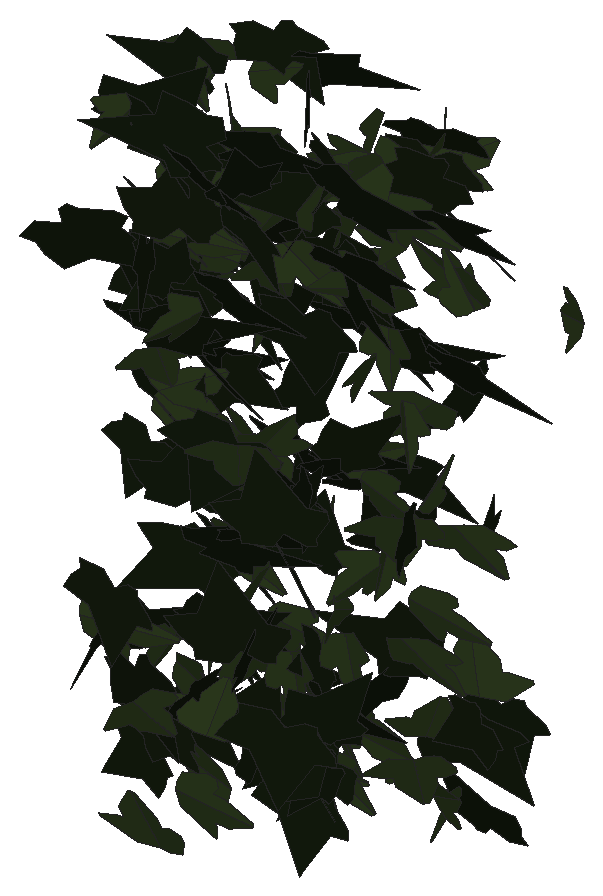
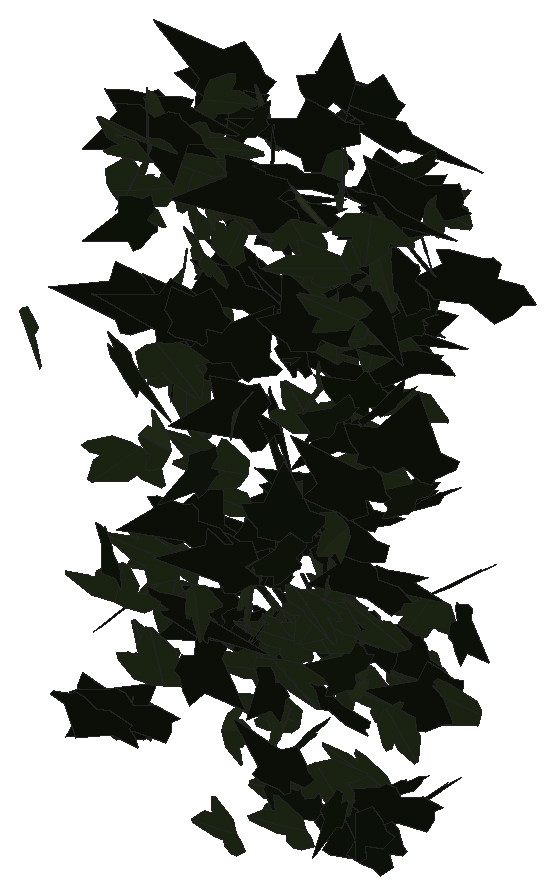
# SketchUp Ruby script. Lengths in millimetres.
U = 1.mm
M = Sketchup.active_model
def pt(a) = Geom::Point3d.new(a.map { |v| v * U })
def face(e, loops, mat)
  f = e.add_face(loops[0].map { |a| pt(a) })
  loops[1..].each { |l| e.add_face(l.map { |a| pt(a) }).erase! }
  f.material = f.back_material = mat if mat
  f
end
# faces: each face lists its corners as indices into pts; further lists are holes
def faces(e, pts, list, mat = nil) = list.each { |f| face(e, (f[0].is_a?(Array) ? f : [f]).map { |l| l.map { |i| pts[i] } }, mat) }
# xy, xz, yz: faces in a plane at the given z, y or x. An outline is a flat list of corners, or four numbers for a rectangle; further outlines are holes
def ring(l) = l.size == 4 ? [[l[0], l[1]], [l[2], l[1]], [l[2], l[3]], [l[0], l[3]]] : l.each_slice(2).to_a
def flat(e, list, mat, &to3) = list.each { |f| face(e, (f[0].is_a?(Array) ? f : [f]).map { |l| ring(l).map { |u, v| to3.(u, v) } }, mat) }
def xy(e, z, list, mat = nil) = flat(e, list, mat) { |x, y| [x, y, z] }
def xz(e, y, list, mat = nil) = flat(e, list, mat) { |x, z| [x, y, z] }
def yz(e, x, list, mat = nil) = flat(e, list, mat) { |y, z| [x, y, z] }
def lines(e, pts, list) = list.each { |a, b| e.add_line(pt(pts[a]), pt(pts[b])) }
# prism: a flat outline (further loops are holes) pulled along v
def prism(e, loops, v, mat = nil)
  f = face(e, loops, mat); d = Geom::Vector3d.new(v.map { |x| x * U })
  f.pushpull(f.normal.samedirection?(d) ? d.length : -d.length)
end
def box(e, o, s, mat = nil) = prism(e, [[o, [o[0] + s[0], o[1], o[2]], [o[0] + s[0], o[1] + s[1], o[2]], [o[0], o[1] + s[1], o[2]]]], [0, 0, s[2]], mat)
def at(x, y, z, deg = 0) = Geom::Transformation.translation(pt([x, y, z])) * Geom::Transformation.rotation(ORIGIN, Z_AXIS, deg.degrees)
def axes(o, x, y, z) = Geom::Transformation.new([*x, 0, *y, 0, *z, 0, *pt(o).to_a, 1])
def part(name) = M.definitions.add(name)
# library, detail: a bought-in or finely detailed component or shape, given as its bounding box
def library(name, o, s) = part(name).tap { |d| box(d.entities, o, s) }
def detail(e, o, s) = box(e.add_group.entities, o, s)
def put(e, d, t, mat = nil) = e.add_instance(d, t).tap { |i| i.material = mat if mat }
def group(e, t, mat = nil) = e.add_group.tap { |g| g.transformation = t; g.material = mat if mat }.entities
root = M.entities
M.materials.add("efeu1").color = [18, 25, 13]
M.materials.add("efeu2").color = [43, 57, 29]
c1 = part("ivyleaf_10")
p = [[0,12.8,-0.8],[-1.5,51.3,-10.9],[-4.9,51,-11.6],[-13.6,26.5,-7.3],[-13.2,15.9,-4.6],[-21.1,19.3,-7.2],
  [-29.5,16.3,-8.3],[-29.2,8.3,-6.2],[-19.7,-9.8,0.5],[-7.6,-13,4],[1,-12.2,5.8],[-0.4,51.1,-11.1],
  [-1.5,51.1,-10.9],[1,-12.4,5.9],[16.9,-12.4,3.5],[35.1,9.1,-5.1],[35,12.9,-6.1],[20.5,16.4,-4.9],
  [15.8,15,-3.8],[15.3,27.6,-7.1],[12.8,31.3,-7.8]]
faces(c1.entities,p,[[0,1,2,3,4,5,6,7,8,9,10],[11,12,0,13,14,15,16,17,18,19,20]],"efeu2")
c2 = part("ivyleaf_9")
p = [[39.1,54.8,31.7],[34.5,51.8,30.2],[-5.3,25.2,17.3],[-17.9,28.3,20.9],[-21.6,21.7,17],[-20.2,4.3,5.3],
  [-22.9,-0.3,2.5],[-17.1,-4,-0.6],[-2,-2.1,-1.2],[-0.7,-15.4,-10.1],[16.6,-22.3,-16.7],[21.1,-15.1,-12.5],
  [32.7,-10.7,-11],[46.1,-1.8,-6.6],[30.8,11.2,3.8]]
faces(c2.entities,p,[[0,1,2,3,4,5,6,7,8,9,10,11,12,13,14]],"efeu1")
put(root,c1,axes([4846,848.6,1966.5],[1.18258,-0.23138,-0.81582],[1.49962,-0.21628,0.66148],[-0.59651,-1.00243,0.04559]))
put(root,c1,axes([4885.7,700.2,2538.1],[-0.36711,-0.69452,0.88742],[0.07213,-0.90382,-0.69911],[2.14348,-0.08853,0.17551]))
put(root,c1,axes([4836.3,714.6,1809.9],[0.3187,-0.20437,-1.17963],[2.21627,-0.24872,0.2084],[-0.52897,-1.16521,0.16242]))
put(root,c2,axes([4878.1,784.3,2193.3],[2.14412,-0.25981,0.56554],[-1.04967,0.1251,1.15616],[-0.5488,-1.25434,-0.00183]))
put(root,c2,axes([4866.7,834.1,1632.7],[0.89169,0.91791,0.16625],[-0.1858,-0.13677,1.03028],[1.76564,-0.47796,0.02446]))
put(root,c2,axes([4851.8,797,2484.4],[0.18117,0.02377,-1.09498],[2.08435,-0.01319,0.09492],[-0.02109,-1.09903,-0.02482]))
put(root,c2,axes([4929.7,790.7,2565.8],[-1.03003,0.34094,0.81684],[-1.45047,0.30741,-0.63327],[-0.85671,-0.93039,0.09008]))
put(root,c1,axes([4893.3,836.9,2570],[-1.65299,-0.58891,-0.0854],[0.14393,0.04063,-1.04933],[1.12335,-0.87177,0.00879]))
put(root,c2,axes([4905,802.3,2267.8],[-0.88881,-0.81019,0.7348],[0.6949,0.63767,0.93514],[-1.96226,0.5928,-0.00167]))
put(root,c2,axes([4867.5,714.2,1803.7],[0.4301,0.19051,1.17744],[1.81265,0.6926,-0.29486],[-1.36655,0.97865,-0.02054]))
put(root,c1,axes([4901.7,773.6,1792.3],[-0.28561,-1.14491,0.34896],[-0.0254,-0.35007,-1.15429],[2.27782,-0.14746,0.03088]))
put(root,c2,axes([4860.8,618.8,2404.9],[0.2146,0.04854,-1.35483],[0.99531,1.25272,0.08841],[2.38046,-0.52816,0.08517]))
put(root,c1,axes([4905.7,792.9,2483.9],[-0.23456,-1.0959,-0.05158],[0.01073,0.05127,-1.10281],[2.088,-0.12337,-0.00013]))
put(root,c2,axes([4897.8,894.6,1717.6],[1.17847,-0.34894,-0.75473],[-1.18072,0.43266,-0.70903],[1.05366,0.87512,0.04961]))
put(root,c2,axes([4899.7,725.4,1645.2],[0.56188,-0.65632,-0.84207],[0.61853,-0.77696,0.71952],[-1.93548,-0.43883,-0.01452]))
put(root,c2,axes([4876.7,763.3,2131],[0.64432,-0.96981,0.40729],[0.38099,-0.36064,-1.02513],[1.96532,0.38786,0.0652]))
put(root,c2,axes([4887.9,782.7,1681.3],[-0.24413,-0.55305,-1.09213],[0.4735,1.06342,-0.56773],[2.28124,-0.27991,0.00096]))
put(root,c2,axes([4915.4,621.2,1867.1],[-0.76393,0.48456,-0.93814],[1.18497,-0.70197,-0.62897],[-1.62302,-0.74058,-0.01765]))
put(root,c2,axes([4881.4,745.3,2394],[1.04099,-0.82406,0.44768],[0.46426,-0.3754,-0.98906],[1.7234,0.59889,-0.00397]))
put(root,c2,axes([4915.5,707.1,2085],[-0.61667,-0.93712,0.43634],[-0.30194,-0.40677,-0.99143],[1.94407,-0.36044,-0.01557]))
put(root,c2,axes([4885.1,861.7,1651],[0.46559,-0.58363,0.86638],[1.32845,-0.5707,-0.58154],[1.47916,0.69626,0.24958]))
put(root,c1,axes([4907.7,796.2,2558.5],[-0.7182,0.19841,-0.94224],[0.76416,-0.88741,-0.34767],[-1.66567,-0.49267,0.24677]))
put(root,c2,axes([4952.8,775.8,2416.3],[0.70779,0.07914,-1.04316],[-1.96269,-0.15844,-0.37967],[-0.33481,1.09607,0.02043]))
put(root,c2,axes([4911.5,740.5,1678.1],[0.52368,-0.71599,-0.67061],[-0.28279,0.65804,-0.76353],[1.8455,0.304,0.0733]))
put(root,c2,axes([4907.6,707.4,2529.9],[-1.02548,-0.17609,1.14757],[2.17278,0.14966,0.559],[-0.40173,1.2589,0.09406]))
put(root,c2,axes([4900.4,816,2023.8],[-0.26356,-0.22747,-1.05466],[1.65883,0.60312,-0.24453],[1.21025,-0.87621,0.10548]))
put(root,c1,axes([4950.4,863.7,1733.6],[-0.95398,-0.91522,0.38623],[-0.31352,-0.35004,-1.04326],[1.86443,-0.52716,0.02219]))
put(root,c2,axes([4927.5,623.3,1922.4],[-0.37026,-1.21348,0.33962],[-0.11374,-0.33437,-1.22896],[2.39553,-0.20343,-0.00586]))
put(root,c1,axes([4940.5,693.8,2224.6],[-1.0711,-0.94475,-0.38083],[0.42097,0.31136,-1.09929],[1.89238,-0.604,0.02899]))
put(root,c2,axes([4910.8,850.8,1893.8],[0.96676,-0.90302,0.37203],[0.34876,-0.32377,-1.03609],[1.82576,0.54001,0.00092]))
put(root,c2,axes([4934.1,729,2314.2],[-1.14695,-0.91496,-0.60108],[0.62428,0.5037,-1.09559],[1.98777,-0.68612,-0.00274]))
put(root,c2,axes([4913,829.8,2149.9],[1.8282,0.40208,-0.31312],[0.55286,0.11694,1.04134],[0.79691,-1.00355,-0.00411]))
put(root,c1,axes([4960.3,886.9,2004.7],[1.67581,-0.45234,-0.39639],[-0.65056,0.20187,-0.98968],[0.94182,0.9443,0.02169]))
put(root,c2,axes([4995,729.9,2335.6],[-1.34925,0.01881,0.95009],[-1.80656,-0.06991,-0.7069],[0.08528,-1.18337,0.05687]))
put(root,c2,axes([4945.7,740,2503.9],[-0.77998,-1.09276,-0.27634],[0.19264,0.25717,-1.16707],[2.13653,-0.42212,0.00435]))
put(root,c1,axes([4974.5,917.2,1908.8],[1.82703,-0.05891,-0.44476],[-0.84624,0.01509,-0.96172],[0.1138,1.05789,-0.01105]))
put(root,c1,axes([4940,824.2,2412],[0.83206,0.37666,-0.93166],[1.36345,0.59568,0.57701],[1.34123,-0.83922,-0.00859]))
put(root,c1,axes([4996.9,735.4,1635.3],[0.10107,-0.03825,-1.11885],[-1.45993,0.81459,-0.06426],[1.55186,0.76883,0.01242]))
put(root,c1,axes([4967.5,727.3,2337.2],[-1.56086,-0.69456,-0.20292],[0.28902,0.13467,-1.07471],[1.34648,-0.83406,-0.00455]))
put(root,c1,axes([4956.2,823.4,2081.1],[-1.21348,0.84104,-0.32874],[0.3791,-0.26153,-1.05541],[-1.67627,-0.66799,-0.0007]))
put(root,c2,axes([4991.7,702.2,2348.9],[-1.84264,-0.54092,0.3383],[-0.52851,-0.19624,-1.10851],[1.09319,-1.00663,0.03431]))
put(root,c2,axes([4998,714.2,1951.4],[-1.9086,-0.47753,0.46517],[-0.77208,-0.22963,-1.11031],[1.0068,-1.08136,0.03037]))
put(root,c2,axes([5007.5,653.9,2303],[0.35354,-0.22916,1.33655],[-1.51332,1.07437,0.29472],[-2.09059,-0.81646,0.01268]))
put(root,c1,axes([4966.9,840.5,1964.7],[-1.62663,-0.48057,-0.40885],[0.65443,0.2224,-0.98024],[1.00683,-0.92096,-0.02338]))
put(root,c1,axes([4941.8,720.7,2167.5],[1.36561,0.02191,-0.77898],[1.47716,0.07501,0.71703],[0.1332,-1.05643,0.03476]))
put(root,c2,axes([4950.5,680.1,2552.1],[0.34669,-1.10973,0.43678],[0.21296,-0.42399,-1.12391],[2.25973,0.21021,0.03891]))
put(root,c1,axes([5010.2,724.9,2370.8],[0.366,0.1832,1.06547],[-1.68571,-0.59383,0.26197],[1.1798,-0.9053,0.04378]))
put(root,c1,axes([4961,738.4,2426.1],[1.79672,0.559,-0.5015],[0.79731,0.27658,1.09691],[1.18623,-1.03259,0.02232]))
put(root,c2,axes([4986.8,921.5,1883],[-0.23289,0.36293,-0.9901],[-1.09432,0.81257,0.36892],[1.68237,0.57879,0.10291]))
put(root,c2,axes([4948.9,642.2,1809.5],[-0.76814,-0.0541,-1.27166],[2.42234,-0.02724,-0.4028],[-0.01832,-1.33389,0.0598]))
put(root,c1,axes([4937.8,733.9,2135.3],[0.76396,0.08272,1.12506],[2.03585,0.35134,-0.40748],[-0.68187,1.14169,0.04388]))
put(root,c2,axes([4960.3,827.1,2243.9],[0.58573,-0.96798,0.36038],[0.29438,-0.3286,-1.01473],[1.94363,0.34148,0.04509]))
put(root,c1,axes([4994.6,788.6,2011.3],[0.25784,-0.62675,-0.90074],[-0.02244,0.90669,-0.63266],[2.08832,0.08713,0.10441]))
put(root,c2,axes([4995.4,766.6,2414.1],[-0.77118,-0.74195,0.67552],[-0.66273,-0.57926,-0.8451],[1.79098,-0.53383,-0.02185]))
put(root,c1,axes([4999.9,760.2,2354.8],[0.05647,0.41781,1.12444],[-0.15753,-1.12139,0.41886],[2.27755,-0.08792,0.00109]))
put(root,c1,axes([4949.4,707.9,2385.3],[0.30934,-0.09909,-1.10519],[2.1095,-0.03787,0.16641],[-0.099,-1.11643,0.09245]))
put(root,c1,axes([4978.2,828.3,1909.9],[-1.79953,-0.23681,0.48641],[0.92969,0.0472,0.97255],[-0.44248,1.06226,0.06522]))
put(root,c1,axes([4962.1,721.4,1776.4],[0.39652,-0.25214,1.07146],[2.0265,-0.23024,-0.26123],[0.531,1.06697,0.19683]))
put(root,c2,axes([5004.9,677.2,2057.4],[-1.86037,-0.16539,0.63639],[1.21591,0.03077,0.98931],[-0.29597,1.16599,0.06416]))
put(root,c2,axes([5052.2,636,2576],[-1.73559,0.24759,0.84965],[-1.58337,0.17617,-0.94427],[-0.57432,-1.23389,0.03567]))
put(root,c2,axes([4994.8,603.5,2425.7],[-0.84423,0.2192,-1.02053],[1.71796,-0.47625,-0.49465],[-0.99755,-1.0057,0.01181]))
put(root,c2,axes([5035.2,597.3,2401.7],[-0.3209,0.63322,0.93226],[-0.59722,0.87898,-0.65379],[-2.06004,-0.35346,0.04432]))
put(root,c1,axes([4980.5,846,2560.2],[0.60133,-0.77769,-0.65248],[1.07239,-0.43408,0.79022],[-1.6071,-0.58064,0.28316]))
put(root,c1,axes([4976.2,817.1,2468.6],[0.49703,0.24354,1.04026],[1.41305,0.72867,-0.35699],[-1.46212,0.787,0.00861]))
put(root,c2,axes([4998,750.4,2190.7],[0.30783,-0.27011,-1.09009],[-0.47582,1.06504,-0.301],[2.08377,0.2831,0.09231]))
put(root,c1,axes([4974.1,889.7,1655.3],[0.6793,-0.12655,0.97045],[1.85458,-0.04987,-0.3649],[0.17278,1.03281,0.10129]))
put(root,c2,axes([4993.7,817.4,2358.6],[1.99773,0.27832,0.13843],[-0.25459,-0.03564,1.08594],[0.53403,-1.05816,-0.00016]))
put(root,c1,axes([5036.1,724.8,2567.2],[-1.09442,0.59245,0.81807],[-1.07705,0.59075,-0.82562],[-1.5923,-0.80679,-0.00381]))
put(root,c2,axes([4996.9,848.7,2616.6],[-0.46448,-0.71089,-0.71488],[0.90752,0.56666,-0.72629],[1.69058,-0.49951,0.19347]))
put(root,c1,axes([5005.5,727.4,1859.2],[0.24641,-0.64646,1.039],[1.00789,-0.9123,-0.63361],[2.09955,0.51382,0.18223]))
put(root,c2,axes([4990.7,860.3,1653.7],[0.36872,-0.66892,0.82761],[0.74126,-0.73828,-0.68789],[1.88475,0.42122,0.10863]))
put(root,c1,axes([5015.4,798.8,2268.4],[-0.10446,0.68257,-0.8647],[0.01922,-0.86542,-0.68378],[-2.09655,-0.04195,0.03681]))
put(root,c2,axes([4989.7,724,2213.9],[0.76092,-0.69204,0.72907],[0.68259,-0.63477,-0.79921],[1.78721,0.53708,-0.00516]))
put(root,c2,axes([4991.4,887,1723.6],[0.06995,-0.09881,1.03993],[1.15812,-0.84377,-0.10168],[1.61596,0.60899,0.02785]))
put(root,c1,axes([4992.1,764.2,1936.8],[1.03645,0.21815,0.87221],[1.54459,0.31953,-0.58665],[-0.73633,0.97735,-0.00289]))
put(root,c1,axes([5022.5,555.3,1824.8],[-1.01623,-0.83901,-0.72053],[0.81293,0.58158,-0.99375],[1.9415,-0.68267,0.03895]))
put(root,c2,axes([5034.5,616.8,2468.8],[-1.62028,-0.53973,0.95737],[1.64347,0.4206,1.00502],[-1.29386,1.21014,0.07768]))
put(root,c1,axes([4995.4,694.8,1629.2],[0.2161,-0.06361,-1.21846],[1.87203,-0.71928,0.12922],[-1.37396,-0.99003,-0.01559]))
put(root,c2,axes([5039.6,633.1,1814.5],[-0.30336,0.30396,-1.08576],[-0.85922,0.98761,0.34276],[1.96633,0.47845,-0.01774]))
put(root,c2,axes([5008.7,720.6,1855.6],[-0.34612,-0.06894,1.01165],[1.86506,-0.27601,0.15735],[0.49581,0.99012,0.11431]))
put(root,c1,axes([5043.6,832.8,1773],[-1.07018,0.99121,0.30142],[-0.29454,0.25875,-1.13958],[-1.94965,-0.58318,0.0067]))
put(root,c2,axes([5033.1,792.7,2314.8],[-0.32139,-0.82216,0.83289],[-0.06191,-0.83789,-0.83369],[2.22649,-0.14197,0.09705]))
put(root,c2,axes([5032.4,832.6,2062.4],[1.89724,-0.49364,-0.00519],[0.05377,0.04537,1.11112],[-0.93801,-0.99585,0.05319]))
put(root,c2,axes([5007.9,615.3,2311.8],[0.79336,0.09656,1.227],[2.25748,0.31422,-0.42771],[-0.62517,1.2572,0.01266]))
put(root,c1,axes([5021.5,713.1,1761.7],[-0.7786,-0.12241,1.15089],[1.7788,-0.75491,0.25194],[1.2992,0.96022,0.34479]))
put(root,c1,axes([5068.1,525.5,1672.7],[-2.16278,0.18281,-0.28609],[-0.53653,0.04886,1.151],[0.36009,1.17083,-0.00336]))
put(root,c2,axes([5008.6,712.4,1969.8],[0.86493,-0.09746,1.03287],[1.95799,-0.10314,-0.4624],[0.25474,1.12371,0.04714]))
put(root,c2,axes([5082,767.6,2499.4],[-1.69453,-0.4522,0.43981],[-0.76257,-0.1822,-0.99846],[0.92727,-0.9762,-0.01738]))
put(root,c2,axes([5018.2,771.5,2080.3],[1.02109,-0.66735,0.79324],[0.99271,-0.59808,-0.85595],[1.70495,0.74791,0.02331]))
put(root,c1,axes([5057.6,770.5,2065.3],[0.79118,-0.94659,0.56429],[0.4029,-0.52327,-1.03375],[2.0583,0.46628,-0.01455]))
put(root,c2,axes([5058.8,715.5,1729.5],[-1.67323,0.64297,0.5186],[0.76141,-0.33117,1.08883],[1.37545,0.9655,0.02812]))
put(root,c1,axes([5073.3,889.4,2247.9],[-0.01998,0.68803,-0.80544],[-0.20061,0.8008,0.68544],[2.00605,0.08694,0.06052]))
put(root,c1,axes([5060.4,641.7,1777.5],[1.2704,0.77562,-0.50549],[0.56457,0.41114,1.02257],[1.66908,-0.72942,0.03886]))
put(root,c2,axes([5033.2,864.7,2576],[1.61987,0.31971,0.86466],[1.54608,0.29622,-0.90918],[-0.82942,1.17657,-0.00606]))
put(root,c2,axes([5050.8,795.9,2288.8],[-0.17066,0.25336,1.0693],[0.44283,-1.04415,0.26691],[2.04401,0.24737,0.03145]))
put(root,c1,axes([5090,844,1961.4],[-0.64932,0.54893,1.02714],[-1.13242,0.83792,-0.64544],[-1.9054,-0.68506,0.03357]))
put(root,c1,axes([5079.4,716.3,1957.1],[0.54915,-1.20887,0.08828],[0.03204,-0.08674,-1.24282],[2.30662,0.28901,-0.00375]))
put(root,c1,axes([5079.9,576.5,2376.7],[0.07404,-0.29592,1.14624],[0.08342,-1.14571,-0.29727],[2.25151,0.05218,-0.02668]))
put(root,c1,axes([5091.2,751.6,2467.5],[-1.05345,-1.04932,0.43132],[-0.30643,-0.4024,-1.18559],[2.13733,-0.57488,0.04261]))
put(root,c1,axes([5072.1,781.4,1627.9],[0.05801,-0.65193,1.0668],[-0.07656,1.06606,0.65262],[-2.3782,-0.05022,0.00501]))
put(root,c1,axes([5079.9,743.7,2372.3],[-1.16177,-0.8753,-0.35463],[0.35219,0.30322,-1.06694],[1.76256,-0.63753,-0.02056]))
put(root,c2,axes([5037.7,691.6,2337.3],[0.86063,-0.3771,0.89753],[1.34392,-0.5542,-0.58862],[1.27547,0.83839,0.0146]))
put(root,c2,axes([5052.9,798.3,1996],[1.36571,-0.84416,-0.05188],[-0.06923,0.03717,-1.10793],[1.60814,0.7185,-0.00363]))
put(root,c1,axes([5046.1,940,1647.3],[0.7237,-0.22211,1.01301],[1.84651,-0.30496,-0.43105],[0.69725,1.03816,0.0901]))
put(root,c2,axes([5066.1,743,1698.2],[1.16904,-0.83268,-0.65475],[-0.59695,0.57996,-1.03181],[1.9256,0.68532,0.07764]))
put(root,c2,axes([5070.4,955.3,2193.3],[1.52334,-0.67234,-0.4119],[-0.57132,0.2829,-1.04509],[1.38763,0.85457,0.0219]))
put(root,c2,axes([5080,700.8,2025],[1.52933,0.83731,0.26818],[0.32261,0.20896,-1.16031],[-1.64192,0.82095,0.02181]))
put(root,c1,axes([5065.7,781.6,1858.1],[-0.4677,-0.01065,-1.02888],[1.86649,-0.32245,-0.2309],[-0.59245,-1.00747,0.08478]))
put(root,c2,axes([5070.9,885.4,2016],[1.15118,0.17213,0.85059],[1.4562,0.38347,-0.6217],[-0.77938,0.97073,0.09477]))
put(root,c2,axes([5112.5,625.9,2188.3],[-2.21542,-0.41683,-0.3484],[0.62378,0.11817,-1.23643],[0.82458,-1.20931,-0.00073]))
put(root,c2,axes([5087,800.7,2591.7],[-0.05634,-0.2082,-1.05353],[1.65292,-0.62454,0.09902],[-1.20215,-0.84896,0.18552]))
put(root,c1,axes([5099.6,705.9,2145],[-0.94528,-0.90904,0.28806],[0.27931,0.24806,1.03583],[-1.79325,0.51782,0.00949]))
put(root,c2,axes([5077.3,590.6,2563.6],[0.64386,-0.60634,0.89815],[1.03125,-0.72019,-0.6903],[1.7861,0.6344,0.07479]))
put(root,c2,axes([5147.8,748.5,2478.3],[-1.14488,-0.20562,0.89498],[-1.41505,-0.51887,-0.61896],[1.02572,-0.94532,0.14506]))
put(root,c2,axes([5088.6,759.9,1957.3],[0.93066,-0.30264,-1.07371],[1.80057,-0.50868,0.57425],[-1.12497,-1.06453,0.03085]))
put(root,c2,axes([5119.9,762,1974.9],[-1.58233,-0.2378,0.72787],[1.37562,0.11101,0.86188],[-0.48115,1.09941,0.07041]))
put(root,c2,axes([5075.5,679.6,2557.4],[1.29871,-0.01309,1.00643],[1.91491,-0.02398,-0.68251],[0.05176,1.21572,-0.00263]))
put(root,c2,axes([5138,820.4,2276],[1.50389,-0.61193,0.69678],[-1.06256,0.41701,0.99938],[-1.40921,-0.96747,-0.00995]))
put(root,c1,axes([5162.2,811.4,2507.3],[0.88105,-0.31074,-0.97167],[-1.58615,0.50017,-0.55701],[1.1197,0.95304,-0.02448]))
put(root,c2,axes([5134.1,717.6,2438.8],[0.25955,0.48472,1.09069],[0.66447,1.03357,-0.50299],[-2.1722,0.37408,-0.02354]))
put(root,c2,axes([5147.9,591.6,1935.6],[-2.18834,-0.33328,0.46317],[0.88319,0.06015,1.1953],[-0.63197,1.23814,0.0666]))
put(root,c2,axes([5152.1,703.8,2078.9],[-0.01238,0.55823,1.15868],[0.0685,1.15832,-0.55786],[-2.44683,0.0296,-0.02148]))
put(root,c2,axes([5138.3,767.4,1834],[-0.37076,-0.26657,1.01239],[-0.75114,-0.93509,-0.32216],[1.84545,-0.43416,0.07227]))
put(root,c1,axes([5143.3,594.4,2200.8],[-1.76311,-0.66734,-0.04645],[0.07345,0.0259,-1.14173],[1.27103,-0.92719,0.00154]))
put(root,c1,axes([5114.4,729.7,1836.9],[1.49222,-0.52836,0.80453],[1.25422,-0.46164,-0.94541],[1.33516,1.02416,-0.01108]))
put(root,c1,axes([5163.3,792.1,1692.3],[-0.59528,0.61221,-0.90819],[-0.75045,0.81822,0.68736],[1.94473,0.50314,-0.01275]))
put(root,c1,axes([5149.3,880.5,1937.1],[-0.13628,-1.03514,-0.23916],[0.08611,0.23651,-1.03723],[2.02014,-0.07991,0.02808]))
put(root,c2,axes([5188.3,762,2381.1],[-1.0651,0.1314,-0.98465],[-1.88368,0.02282,0.56558],[0.16155,1.13234,0.10286]))
put(root,c1,axes([5140.3,864.7,2536.8],[0.35009,-0.86556,0.7367],[0.62857,-0.67338,-0.87363],[2.06988,0.35088,0.1407]))
put(root,c2,axes([5149.5,590.6,1902.2],[0.12855,0.20457,1.36192],[0.99578,1.25751,-0.21483],[-2.42456,0.52731,-0.01602]))
put(root,c1,axes([5152.9,809.6,2431],[-0.3634,-0.65608,-0.90815],[-0.42655,-0.88026,0.68305],[-2.08915,0.29385,0.01851]))
put(root,c2,axes([5149,592.7,2565.2],[0.94114,0.60468,0.84448],[-1.26263,-0.53575,0.77211],[1.52095,-0.81893,0.11842]))
put(root,c2,axes([5125.6,784.1,2400.7],[-0.60269,-0.24893,-1.15327],[1.99183,0.49202,-0.39358],[1.03669,-1.09006,0.08572]))
put(root,c2,axes([5177.9,587,1785.4],[0.01339,0.47244,1.11694],[-0.08482,1.11631,-0.47189],[-2.30655,-0.03831,0.02384]))
put(root,c1,axes([5124.9,729.4,1701.2],[-0.22611,-0.0745,1.02824],[1.70174,0.50776,0.1401],[-0.97665,0.90199,0.00606]))
put(root,c1,axes([5149.2,810.7,2098.8],[-0.13344,-0.37064,1.08543],[0.61764,1.03661,0.37493],[-2.0937,0.32942,0.04142]))
put(root,c2,axes([5196,664.1,2114.6],[0.03934,0.01104,-1.3144],[-2.28038,0.5407,-0.0143],[1.02867,1.19821,0.01856]))
put(root,c2,axes([5183.4,609.8,1771.3],[-1.28177,0.8523,-0.68627],[-0.79591,0.54418,1.08624],[1.92447,0.79272,-0.00784]))
put(root,c2,axes([5157.2,704.2,2342.1],[-1.57527,-0.27917,-0.92575],[1.66644,0.30058,-0.8735],[0.78071,-1.20488,-0.00342]))
put(root,c2,axes([5149.4,602,2517.4],[0.39911,-1.05024,0.41894],[0.23494,-0.40227,-1.07025],[2.13911,0.24013,0.03938]))
put(root,c2,axes([5145.1,889.4,2057.8],[-0.11966,-0.11772,-1.07569],[1.42154,0.77493,-0.12846],[1.49018,-0.74869,0.03617]))
put(root,c2,axes([5149.5,784.3,2366.7],[-0.73359,-0.24415,-1.10407],[1.83986,0.53392,-0.45557],[1.11632,-1.04042,0.02531]))
put(root,c1,axes([5150.6,695,2430.4],[1.48435,0.36089,0.74312],[1.2369,0.36287,-0.85831],[-0.97062,1.01432,0.04266]))
put(root,c1,axes([5180.2,661.1,1794.2],[-0.68254,-0.88225,-0.74204],[0.62048,0.66778,-0.95152],[2.10448,-0.48303,0.03988]))
put(root,c2,axes([5194,824.4,1805.4],[-0.65528,0.66889,-1.08885],[0.94373,-0.96939,-0.7523],[-2.24152,-0.60368,0.00158]))
put(root,c2,axes([5170.8,676.8,2243.2],[-0.67009,1.08034,0.65143],[0.29311,-0.63446,1.13543],[2.38301,0.38182,0.04352]))
put(root,c2,axes([5192.4,836.6,1996.7],[1.06448,0.35477,1.03144],[-1.65329,-0.55611,0.66233],[1.25541,-1.03317,-0.00233]))
put(root,c2,axes([5239,819.1,1859.4],[-1.21288,0.38851,0.94094],[-1.54892,0.47241,-0.74627],[-1.16385,-1.0336,0.0126]))
put(root,c2,axes([5168.2,729.9,2140.9],[1.35753,0.48201,0.85894],[1.37196,0.46718,-0.8608],[-1.27735,1.01405,-0.0117]))
put(root,c1,axes([5199.7,710.8,1955.4],[0.14084,-0.65887,-1.06764],[0.18092,1.06937,-0.65335],[2.38085,-0.04228,0.11281]))
put(root,c1,axes([5192.3,666.2,2526],[0.65303,-1.07913,-0.40514],[0.33312,-0.36903,1.13118],[-2.16833,-0.38169,0.05177]))
put(root,c2,axes([5183.1,665.8,1774.9],[-0.4758,0.02469,-1.05952],[2.01585,-0.03135,-0.25066],[-0.06887,-1.08816,-0.01682]))
put(root,c2,axes([5189.6,726.7,2555.4],[0.07985,-0.81298,0.81091],[0.22501,-0.80408,-0.81225],[2.17376,0.11309,0.05429]))
put(root,c1,axes([5241.4,781.2,2540.6],[0.18022,0.11164,1.21981],[-1.31011,-1.00712,0.14561],[1.92828,-0.69469,-0.01508]))
put(root,c2,axes([5207.1,699,1811.4],[0.34982,-0.2267,-1.04176],[-0.72021,0.97442,-0.27881],[1.89696,0.41176,0.08625]))
put(root,c1,axes([5242,636.8,1720.5],[-1.1305,0.69191,-0.71844],[-0.89747,0.54203,0.9119],[1.67279,0.75841,0.00371]))
put(root,c1,axes([5228.7,746.1,2005.3],[-0.37235,-0.67296,1.01536],[-0.07885,-1.02411,-0.68673],[2.317,-0.143,0.1398]))
put(root,c1,axes([5203.3,796,2396.8],[1.494,-0.50136,0.6475],[1.02437,-0.36012,-0.93137],[1.17463,0.95173,-0.01132]))
put(root,c1,axes([5186.5,701.9,1738.5],[1.07536,-0.02066,0.98754],[1.87835,-0.03441,-0.56541],[0.07637,1.13724,0.00083]))
put(root,c2,axes([5190.1,815.1,2304.3],[0.4139,-0.4109,0.99451],[1.17938,-0.78166,-0.45847],[1.67426,0.6522,0.0771]))
put(root,c1,axes([5236.9,729.8,2299.4],[0.25685,-1.23518,-0.02098],[0.00024,0.02112,-1.24253],[2.35113,0.13494,0.00242]))
put(root,c1,axes([5203.2,786.6,2087.4],[-0.20355,0.14783,-1.10289],[1.5508,-0.74414,-0.17876],[-1.44225,-0.82101,-0.03656]))
put(root,c1,axes([5242,770.4,2499.1],[-1.31341,-0.76058,-0.31741],[0.38988,0.2427,-1.02694],[1.5193,-0.71979,-0.01087]))
put(root,c1,axes([5217.8,705.3,1909.4],[1.50291,-0.48284,0.76635],[1.24222,-0.40159,-0.92559],[1.19525,1.0245,-0.00164]))
put(root,c2,axes([5225.1,694.5,2181.7],[-0.29157,-0.07308,1.12984],[1.83561,0.58873,0.16886],[-1.1286,0.97643,-0.01726]))
put(root,c2,axes([5236.9,610.9,1747.7],[-0.59141,-1.22417,0.26123],[-0.11918,-0.25361,-1.263],[2.37932,-0.31699,0.00167]))
put(root,c1,axes([5259.6,711.1,2578.7],[0.36885,0.4703,-1.1324],[-1.00971,-1.00142,-0.5067],[-2.1039,0.56306,0.04465]))
put(root,c2,axes([5266.8,524.6,2167.4],[-2.12474,-0.28305,0.34904],[0.64237,0.08897,1.15172],[-0.56466,1.1663,-0.00315]))
put(root,c1,axes([5273.2,792.7,2222.3],[-1.42065,-0.63996,0.55279],[-0.71359,-0.41045,-0.98146],[1.4426,-0.83325,0.0589]))
put(root,c1,axes([5296.1,690.3,2441.3],[-0.93807,-0.29297,1.13506],[-1.86306,-0.57454,-0.57338],[1.22741,-1.09599,-0.00284]))
put(root,c2,axes([5224.4,711.8,1809.7],[2.15822,-0.14508,0.1181],[0.22347,-0.01282,-1.14323],[0.27715,1.14005,0.00217]))
put(root,c2,axes([5268.1,819.8,2590.1],[1.10479,0.6413,-0.62546],[-0.84124,-0.4432,-0.86466],[-1.4829,0.72921,0.02454]))
put(root,c2,axes([5265.7,914.1,1975.7],[0.10007,0.34053,1.03455],[0.32497,1.02037,-0.34454],[-2.04725,0.17861,-0.00412]))
put(root,c2,axes([5273,606.5,1802.8],[-1.7249,0.48453,-0.55537],[0.87121,-0.31982,-1.02605],[-1.09935,-1.01368,0.05826]))
put(root,c1,axes([5260.4,820.6,1758.9],[-1.55493,-0.78336,0.02363],[0.06987,-0.00416,1.13153],[-1.48993,0.81734,0.0284]))
put(root,c2,axes([5270,622.7,1802.3],[-0.80584,-0.74785,0.71431],[-0.71744,-0.60715,-0.85911],[1.83283,-0.56647,-0.02223]))
put(root,c2,axes([5251.2,614.4,1852],[-0.72312,-0.22674,1.07804],[1.86725,0.44898,0.44022],[-0.95352,1.05117,0.04451]))
put(root,c1,axes([5300.6,704.9,1791.3],[0.40429,-0.21413,-1.11299],[-1.52105,0.77463,-0.30157],[1.52953,0.82694,-0.00571]))
put(root,c1,axes([5271.3,804.6,2088.9],[0.53421,-0.75968,0.88908],[-0.51173,0.84791,0.80939],[-2.16604,-0.38768,0.02805]))
put(root,c2,axes([5234.5,789.8,2286.1],[0.80312,0.05857,1.04073],[1.94839,0.18805,-0.42568],[-0.37341,1.10717,0.01724]))
put(root,c2,axes([5233.6,684,2433],[0.50434,-0.18663,-1.27978],[2.37572,-0.30487,0.30293],[-0.64397,-1.27088,0.11527]))
put(root,c1,axes([5288.1,733,2492.3],[-0.44171,-0.41819,-1.13662],[-0.98702,-1.01152,0.47806],[-2.08297,0.56799,0.01451]))
put(root,c2,axes([5270.7,523.6,1891.9],[-1.22205,-1.04679,-0.25794],[0.24796,0.22268,-1.22802],[2.03681,-0.65516,-0.00526]))
put(root,c2,axes([5273.9,803.1,2560.6],[-1.45178,-0.68855,-0.51611],[0.74163,0.33852,-1.02757],[1.46015,-0.85653,0.00877]))
put(root,c1,axes([5289.7,802.3,2601.2],[0.13287,-0.93094,-0.81556],[-0.07354,0.81482,-0.9334],[2.35435,0.07799,0.01687]))
put(root,c2,axes([5258.5,855.6,2458.3],[1.68593,-0.62923,-0.08232],[-0.11871,0.05434,-1.08654],[1.2019,0.88799,0.00816]))
put(root,c2,axes([5316.7,764.8,2566.8],[-0.27293,-0.27349,-1.03819],[-0.79786,-0.94999,0.30817],[-1.88108,0.44262,0.01993]))
put(root,c2,axes([5306.5,850.1,2237.9],[-1.62958,0.78935,-0.53568],[0.75852,-0.35798,-1.16454],[-1.64952,-0.94442,-0.0063]))
put(root,c2,axes([5262.3,880.1,1734.5],[-0.59114,-0.51139,-1.10038],[1.03321,0.95727,-0.59812],[2.06534,-0.62525,-0.01573]))
put(root,c2,axes([5278,934.5,1746.4],[-1.27696,-0.28649,-0.81053],[1.42177,0.31448,-0.72955],[0.80962,-1.00411,0.00277]))
put(root,c1,axes([5289.9,703.8,2062.7],[0.06241,0.69958,-0.9135],[-0.15417,-0.9102,-0.69996],[-2.1844,0.08423,0.0233]))
put(root,c1,axes([5258.5,817,1930.1],[-0.29123,0.10894,-1.11588],[1.89779,-0.50166,-0.18572],[-0.97555,-1.00844,-0.02816]))
put(root,c1,axes([5268.5,827.9,2545.6],[1.57772,0.01678,-0.80073],[1.47217,0.28198,0.80673],[0.39515,-1.11752,0.19153]))
put(root,c1,axes([5286.1,758.4,1907.5],[-1.65661,0.13392,-0.62445],[1.17583,-0.09087,-0.88067],[-0.30794,-1.0674,-0.00337]))
put(root,c1,axes([5303,809.5,1681.7],[0.4679,-0.65126,0.83246],[0.46657,-0.79624,-0.69532],[1.95672,0.34559,-0.03327]))
put(root,c2,axes([5262.1,649.1,2568.4],[0.46461,-0.25417,1.2546],[1.73897,-0.85991,-0.352],[1.70627,0.9456,0.01713]))
put(root,c1,axes([5300.1,684.1,2373.2],[1.56609,-0.508,0.51793],[0.81587,-0.29134,-0.96684],[1.11388,0.92762,-0.02003]))
put(root,c1,axes([5282.6,728.6,2521.6],[-0.41055,-0.05911,-1.08823],[1.90565,-0.44876,-0.17411],[-0.81896,-1.01459,0.14041]))
put(root,c1,axes([5329.4,677.6,2128],[-1.69109,-0.87624,-0.0737],[0.10621,0.04837,-1.24792],[1.67018,-0.89029,0.00474]))
put(root,c2,axes([5308.8,595.5,2525.4],[2.10992,0.29189,-0.22986],[-0.42114,-0.06232,-1.14639],[-0.56799,1.13048,-0.00385]))
put(root,c1,axes([5364.2,759.9,2425.5],[-1.30881,0.32757,-0.98954],[-1.69437,0.432,0.76171],[1.03179,1.12494,-0.00437]))
put(root,c2,axes([5350,821,1660],[0.94715,-0.53713,0.87346],[-1.15801,0.62681,0.73212],[-1.57084,-0.78594,-0.01305]))
put(root,c1,axes([5332.3,820.7,1850.6],[2.22841,0.29132,0.10886],[-0.20755,-0.01252,1.20649],[0.55429,-1.17586,0.01412]))
put(root,c1,axes([5324.7,803.9,2058.6],[-1.83036,-0.2443,-0.53757],[1.01732,0.07633,-0.99098],[0.47748,-1.09913,0.05066]))
put(root,c1,axes([5341.1,688.8,1795.4],[-1.53411,-0.88088,-0.24425],[0.31546,0.1794,-1.19403],[1.71091,-0.82293,0.00115]))
put(root,c1,axes([5321.6,754.1,1716.8],[-1.36721,0.20874,0.84062],[1.38325,-0.4488,0.73255],[0.89669,1.01059,0.15169]))
put(root,c1,axes([5336.2,681.5,2280.4],[-0.12169,1.06124,-0.60286],[0.03311,-0.60283,-1.06304],[-2.32266,-0.06419,0.01643]))
put(root,c2,axes([5303.9,797.8,2286.8],[1.62957,-0.37304,0.70548],[1.21964,-0.29525,-0.93389],[0.90516,1.06942,-0.01174]))
put(root,c2,axes([5349.7,801.1,1807.1],[0.55509,-0.70234,-0.78555],[0.60227,-0.71908,0.7604],[-1.91291,-0.43021,0.01145]))
put(root,c2,axes([5321.5,726.4,2526.6],[2.11683,0.3174,0.36285],[0.66862,0.09115,-1.15662],[-0.62829,1.16638,-0.00835]))
put(root,c1,axes([5359.9,761,2419.2],[-0.29391,1.23428,0.10625],[0.02455,-0.10547,1.2439],[2.35764,0.15497,0.00029]))
put(root,c2,axes([5365.2,637.1,2148.8],[0.23117,-0.14507,-1.19635],[-1.64668,0.82649,-0.18806],[1.59653,0.87345,-0.02075]))
put(root,c1,axes([5374.6,956,2307],[0.41354,-0.55686,-0.98749],[-0.64015,0.92853,-0.59762],[2.06048,0.40024,0.01252]))
